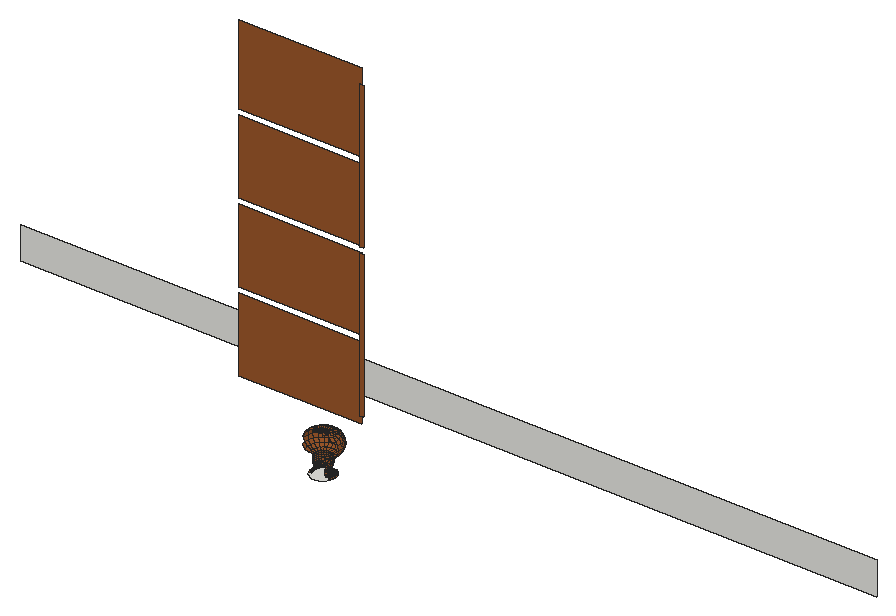
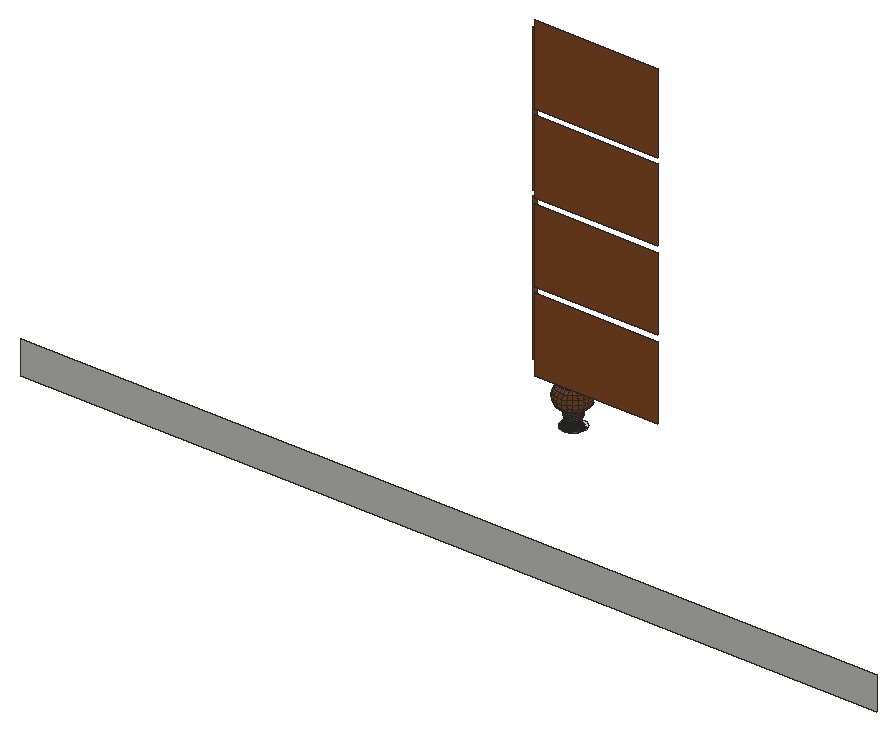
# SketchUp Ruby script. Lengths in inches.
U = 1.inch
M = Sketchup.active_model
def pt(a) = Geom::Point3d.new(a.map { |v| v * U })
def face(e, loops, mat)
  f = e.add_face(loops[0].map { |a| pt(a) })
  loops[1..].each { |l| e.add_face(l.map { |a| pt(a) }).erase! }
  f.material = f.back_material = mat if mat
  f
end
# faces: each face lists its corners as indices into pts; further lists are holes
def faces(e, pts, list, mat = nil) = list.each { |f| face(e, (f[0].is_a?(Array) ? f : [f]).map { |l| l.map { |i| pts[i] } }, mat) }
# xy, xz, yz: faces in a plane at the given z, y or x. An outline is a flat list of corners, or four numbers for a rectangle; further outlines are holes
def ring(l) = l.size == 4 ? [[l[0], l[1]], [l[2], l[1]], [l[2], l[3]], [l[0], l[3]]] : l.each_slice(2).to_a
def flat(e, list, mat, &to3) = list.each { |f| face(e, (f[0].is_a?(Array) ? f : [f]).map { |l| ring(l).map { |u, v| to3.(u, v) } }, mat) }
def xy(e, z, list, mat = nil) = flat(e, list, mat) { |x, y| [x, y, z] }
def xz(e, y, list, mat = nil) = flat(e, list, mat) { |x, z| [x, y, z] }
def yz(e, x, list, mat = nil) = flat(e, list, mat) { |y, z| [x, y, z] }
def lines(e, pts, list) = list.each { |a, b| e.add_line(pt(pts[a]), pt(pts[b])) }
# prism: a flat outline (further loops are holes) pulled along v
def prism(e, loops, v, mat = nil)
  f = face(e, loops, mat); d = Geom::Vector3d.new(v.map { |x| x * U })
  f.pushpull(f.normal.samedirection?(d) ? d.length : -d.length)
end
def box(e, o, s, mat = nil) = prism(e, [[o, [o[0] + s[0], o[1], o[2]], [o[0] + s[0], o[1] + s[1], o[2]], [o[0], o[1] + s[1], o[2]]]], [0, 0, s[2]], mat)
def at(x, y, z, deg = 0) = Geom::Transformation.translation(pt([x, y, z])) * Geom::Transformation.rotation(ORIGIN, Z_AXIS, deg.degrees)
def axes(o, x, y, z) = Geom::Transformation.new([*x, 0, *y, 0, *z, 0, *pt(o).to_a, 1])
def part(name) = M.definitions.add(name)
# library, detail: a bought-in or finely detailed component or shape, given as its bounding box
def library(name, o, s) = part(name).tap { |d| box(d.entities, o, s) }
def detail(e, o, s) = box(e.add_group.entities, o, s)
def put(e, d, t, mat = nil) = e.add_instance(d, t).tap { |i| i.material = mat if mat }
def group(e, t, mat = nil) = e.add_group.tap { |g| g.transformation = t; g.material = mat if mat }.entities
root = M.entities
M.materials.add("[Wood Cherry Original]").color = [152, 86, 42]
xy(root,6,[[197.18,64.59,197.74,64.59,198.28,64.73,198.76,65.01,199.16,65.4,199.4375,65.89,199.59,66.42,199.59,66.98,199.44,67.52,199.17,68.01,198.77,68.4,198.29,68.69,197.75,68.83,197.19,68.83,196.65,68.69,196.17,68.41,195.77,68.02,195.49,67.54,195.35,67,195.34,66.44,195.49,65.9,195.76,65.42,196.16,65.02,196.64,64.74]])
xy(root,6,[[199.4375,65.89,199.59,66.42,199.44,66.45,199.3,65.94],[195.49,65.9,195.625,65.96,195.49,66.46,195.34,66.44],[199.59,66.42,199.59,66.98,199.4375,66.96,199.44,66.45],[195.34,66.44,195.49,66.46,195.5,66.98,195.35,67],[199.4375,66.96,199.59,66.98,199.44,67.52,199.3,67.47],
  [195.5,66.98,195.63,67.48,195.49,67.54,195.35,67],[199.3,67.47,199.44,67.52,199.17,68.01,199.05,67.92],[195.63,67.48,195.89,67.93,195.77,68.02,195.49,67.54],[199.05,67.92,199.17,68.01,198.77,68.4,198.68,68.28],[195.89,67.93,196.26,68.29,196.17,68.41,195.77,68.02],
  [198.68,68.28,198.77,68.4,198.29,68.69,198.23,68.55],[196.26,68.29,196.71,68.55,196.65,68.69,196.17,68.41],[196.71,68.55,197.21,68.68,197.19,68.83,196.65,68.69],[198.23,68.55,198.29,68.69,197.75,68.83,197.73,68.68],[197.21,68.68,197.73,68.68,197.75,68.83,197.19,68.83]],"[Wood Cherry Original]")
xz(root,67.9,[[197.3125,6.79,197.63,6.94]],"[Wood Cherry Original]")
xz(root,68.21,[[197.27,8.1,197.67,8.4]],"[Wood Cherry Original]")
xz(root,69.11,[[202.15,16.08,202.9,42.58],[202.15,43.58,202.9,70.08]],"[Wood Cherry Original]")
xz(root,70.11,[[179.35,14.08,201.81,27.58],[179.35,28.58,201.81,42.08],[179.35,43.08,201.81,56.58],[179.35,57.58,201.81,72.08]],"[Wood Cherry Original]")
xz(root,96.25,[[118.75,0,274.48,6]])
yz(root,195.97,[[66.52,8.1,66.52,8.4,66.92,8.4,66.91,8.1]],"[Wood Cherry Original]")
yz(root,196.27,[[66.56,6.79,66.875,6.94]],"[Wood Cherry Original]")
yz(root,198.66,[[66.55,6.79,66.86,6.94]],"[Wood Cherry Original]")
yz(root,198.96,[[66.51,8.1,66.9,8.4]],"[Wood Cherry Original]")
p = [[199.16,66,6.03],[199.3,65.94,6],[199.44,66.45,6],[199.29,66.47,6.03],[195.64,66.48,6.03],[195.49,66.46,6],
  [195.625,65.96,6],[195.76,66.02,6.03],[195.78,66.5,6.08],[195.9,66.07,6.08],[199.03,66.06,6.08],[199.15,66.48,6.08],
  [199.4375,66.96,6],[199.29,66.95,6.03],[195.64,66.96,6.03],[195.5,66.98,6],[195.78,66.94,6.08],[199.15,66.93,6.08],
  [195.9,67.37,6.08],[195.77,67.42,6.03],[199.17,67.41,6.03],[199.04,67.36,6.08],[199.3,67.47,6],[195.63,67.48,6],
  [196.01,67.84,6.03],[195.89,67.93,6],[196.125,67.75,6.08],[198.93,67.83,6.03],[198.82,67.74,6.08],[199.05,67.92,6],
  [198.59,68.17,6.03],[198.5,68.05,6.08],[196.35,68.18,6.03],[196.26,68.29,6],[196.4375,68.0625,6.08],[198.68,68.28,6],
  [196.82,68.28,6.08],[196.77,68.41,6.03],[198.18,68.41,6.03],[198.12,68.28,6.08],[196.71,68.55,6],[198.23,68.55,6],
  [197.25,68.4,6.08],[197.23,68.54,6.03],[197.71,68.53,6.03],[197.69,68.39,6.08],[197.21,68.68,6],[197.73,68.68,6],
  [195.91,66.51,6.16],[196.02,66.12,6.16],[198.91,66.11,6.16],[199.02,66.5,6.16],[195.91,66.92,6.16],[199.02,66.91,6.16],
  [196.02,67.32,6.16],[198.91,67.31,6.16],[196.23,67.67,6.16],[198.71,67.66,6.16],[196.52,67.96,6.16],[198.42,67.95,6.16],
  [196.87,68.16,6.16],[198.07,68.16,6.16],[197.27,68.27,6.16],[197.68,68.26,6.16],[196.125,66.16,6.25],[196.22,65.76,6.16],
  [196.3125,65.83,6.25],[196.03,66.53,6.25],[198.8,66.15,6.25],[198.9,66.52,6.25],[196.03,66.91,6.25],[198.9,66.9,6.25],
  [196.13,67.27,6.25],[198.81,67.26,6.25],[196.32,67.6,6.25],[198.62,67.59,6.25],[196.59,67.87,6.25],[198.35,67.86,6.25],
  [196.92,68.05,6.25],[198.03,68.05,6.25],[197.28,68.15,6.25],[197.66,68.15,6.25],[196.21,66.2,6.37],[196.39,65.89,6.37],
  [198.54,65.88,6.37],[198.61,65.82,6.25],[198.71,66.1875,6.37],[196.12,66.54,6.37],[198.81,66.53,6.37],[196.125,66.89,6.37],
  [198.81,66.88,6.37],[196.22,67.24,6.37],[198.72,67.23,6.37],[196.39,67.54,6.37],[198.54,67.53,6.37],[196.65,67.79,6.37],
  [198.29,67.78,6.37],[196.95,67.97,6.37],[197.99,67.96,6.37],[197.29,68.06,6.37],[197.65,68.05,6.37],[196.28,66.23,6.5],
  [196.45,65.9375,6.5],[198.48,65.93,6.5],[198.65,66.22,6.5],[196.2,66.55,6.5],[198.73,66.54,6.5],[196.2,66.88,6.5],
  [198.73,66.875,6.5],[196.29,67.21,6.5],[198.65,67.2,6.5],[196.45,67.49,6.5],[198.48,67.49,6.5],[196.69,67.73,6.5],
  [198.25,67.72,6.5],[196.98,67.9,6.5],[197.96,67.89,6.5],[197.3,67.98,6.5],[197.64,67.98,6.5],[196.33,66.25,6.64],
  [196.49,65.97,6.64],[198.4375,65.96,6.64],[198.6,66.24,6.64],[196.25,66.56,6.64],[198.68,66.55,6.64],[198.68,66.87,6.64],
  [196.25,66.88,6.64],[196.33,67.1875,6.64],[198.6,67.18,6.64],[196.49,67.46,6.64],[198.44,67.46,6.64],[196.72,67.6875,6.64],
  [198.22,67.68,6.64],[197,67.85,6.64],[197.94,67.84,6.64],[197.31,67.93,6.64],[197.63,67.93,6.64],[196.35,66.26,6.79],
  [196.51,65.98,6.79],[198.42,65.98,6.79],[198.57,66.25,6.79],[196.27,66.56,6.79],[198.66,66.55,6.79],[198.66,66.86,6.79],
  [196.27,66.875,6.79],[196.36,67.18,6.79],[198.58,67.17,6.79],[196.51,67.45,6.79],[198.42,67.44,6.79],[196.74,67.67,6.79],
  [198.2,67.66,6.79],[197.01,67.82,6.79],[197.93,67.82,6.79],[197.3125,67.9,6.79],[197.63,67.9,6.79],[196.35,66.26,6.94],
  [196.51,65.98,6.94],[198.42,65.98,6.94],[198.57,66.25,6.94],[198.66,66.55,6.94],[196.27,66.56,6.94],[196.36,67.18,6.94],
  [196.27,66.875,6.94],[198.66,66.86,6.94],[198.58,67.17,6.94],[196.51,67.45,6.94],[198.42,67.44,6.94],[196.74,67.67,6.94],
  [198.2,67.66,6.94],[197.01,67.82,6.94],[197.93,67.82,6.94],[197.3125,67.9,6.94],[197.63,67.9,6.94],[196.33,66.25,7.09],
  [196.49,65.97,7.09],[198.4375,65.96,7.09],[198.6,66.24,7.09],[196.25,66.56,7.09],[198.68,66.55,7.09],[198.68,66.87,7.09],
  [196.25,66.88,7.09],[196.33,67.1875,7.09],[198.6,67.18,7.09],[196.49,67.46,7.09],[198.44,67.46,7.09],[196.72,67.69,7.09],
  [198.22,67.68,7.09],[197,67.85,7.09],[197.94,67.85,7.09],[197.31,67.93,7.09],[197.63,67.93,7.09],[196.28,66.23,7.23],
  [196.45,65.9375,7.23],[198.48,65.93,7.23],[198.65,66.22,7.23],[196.2,66.55,7.23],[198.73,66.54,7.23],[196.2,66.88,7.23],
  [198.74,66.875,7.23],[196.28,67.21,7.23],[198.65,67.2,7.23],[196.45,67.5,7.23],[198.48,67.49,7.23],[196.69,67.73,7.23],
  [198.25,67.72,7.23],[196.98,67.9,7.23],[197.96,67.89,7.23],[197.3,67.98,7.23],[197.64,67.98,7.23],[196.18,66.18,7.51],
  [196.36,65.87,7.51],[198.57,65.86,7.51],[198.75,66.17,7.51],[196.09,66.54,7.51],[198.84,66.53,7.51],[196.09,66.9,7.51],
  [198.85,66.89,7.51],[196.18,67.25,7.51],[198.75,67.24,7.51],[196.36,67.5625,7.51],[198.57,67.55,7.51],[196.62,67.82,7.51],
  [198.32,67.8125,7.51],[196.9375,68,7.51],[198,68,7.51],[197.29,68.09,7.51],[197.65,68.09,7.51],[196.11,66.16,7.8],
  [196.3,65.82,7.8],[198.625,65.8125,7.8],[198.82,66.15,7.8],[198.92,66.51,7.8],[196.01,66.53,7.8],[196.01,66.91,7.8],
  [198.92,66.9,7.8],[196.11,67.28,7.8],[198.82,67.27,7.8],[196.3,67.61,7.8],[198.63,67.6,7.8],[196.58,67.88,7.8],
  [198.36,67.87,7.8],[196.91,68.07,7.8],[198.03,68.07,7.8],[197.28,68.17,7.8],[197.66,68.17,7.8],[196.07,66.14,8.1],
  [196.27,65.8,8.1],[198.66,65.79,8.1],[198.86,66.13,8.1],[195.97,66.52,8.1],[198.96,66.51,8.1],[195.97,66.91,8.1],
  [198.96,66.9,8.1],[196.08,67.29,8.1],[198.86,67.28,8.1],[196.27,67.63,8.1],[198.66,67.625,8.1],[196.55,67.91,8.1],
  [198.39,67.9,8.1],[196.89,68.11,8.1],[198.05,68.1,8.1],[197.27,68.21,8.1],[197.67,68.21,8.1],[195.97,66.52,8.4],
  [196.07,66.14,8.4],[198.86,66.13,8.4],[198.96,66.51,8.4],[196.07,67.3,8.4],[195.97,66.92,8.4],[198.96,66.9,8.4],
  [198.86,67.28,8.4],[196.27,67.64,8.4],[198.67,67.625,8.4],[196.55,67.91,8.4],[198.39,67.91,8.4],[196.89,68.11,8.4],
  [198.05,68.11,8.4],[197.27,68.21,8.4],[197.67,68.21,8.4],[196.1,66.15,8.7],[196.26,65.8,8.4],[196.29,65.82,8.7],
  [196,66.53,8.7],[198.83,66.14,8.7],[198.93,66.51,8.7],[196,66.91,8.7],[198.93,66.9,8.7],[196.1,67.28,8.7],
  [198.83,67.27,8.7],[196.3,67.62,8.7],[198.64,67.61,8.7],[196.57,67.89,8.7],[198.37,67.88,8.7],[196.91,68.08,8.7],
  [198.04,68.07,8.7],[197.28,68.18,8.7],[197.66,68.17,8.7],[196.16,66.18,8.99],[196.35,65.86,8.99],[198.58,65.85,8.99],
  [198.63,65.81,8.7],[198.76,66.17,8.99],[198.86,66.52,8.99],[196.07,66.53,8.99],[196.07,66.9,8.99],[198.86,66.89,8.99],
  [196.17,67.26,8.99],[198.77,67.24,8.99],[198.58,67.5625,8.99],[196.35,67.57,8.99],[196.61,67.83,8.99],[198.33,67.82,8.99],
  [196.93,68.01,8.99],[198.01,68.01,8.99],[197.29,68.11,8.99],[197.65,68.1,8.99],[195.375,66.45,9.21],[195.52,65.91,9.21],
  [199.41,65.9,9.21],[199.55,66.43,9.21],[195.375,67,9.21],[199.56,66.98,9.21],[195.52,67.53,9.21],[199.42,67.51,9.21],
  [199.14,67.99,9.21],[195.8,68,9.21],[196.1875,68.39,9.21],[198.76,68.38,9.21],[196.67,68.66,9.21],[198.28,68.66,9.21],
  [197.2,68.8,9.21],[197.75,68.8,9.21],[194.8,66.37,9.66],[194.98,65.69,9.66],[199.94,65.67,9.66],[200.13,66.35,9.66],
  [194.8,67.07,9.66],[200.13,67.05,9.66],[194.99,67.75,9.66],[199.95,67.73,9.66],[195.34,68.36,9.66],[199.6,68.34,9.66],
  [195.84,68.85,9.66],[199.11,68.84,9.66],[196.45,69.2,9.66],[198.5,69.19,9.66],[197.125,69.38,9.66],[197.83,69.375,9.66],
  [194.42,66.32,10.28],[194.63,65.55,10.28],[194.43,67.125,10.28],[200.51,66.3,10.28],[200.51,67.1,10.28],[194.64,67.9,10.28],
  [200.3,67.875,10.28],[195.04,68.59,10.28],[199.91,68.57,10.28],[199.34,69.14,10.28],[195.61,69.15,10.28],[198.65,69.54,10.28],
  [196.3,69.55,10.28],[197.08,69.75,10.28],[197.88,69.75,10.28],[194.29,67.14,11],[194.29,66.31,11],[200.64,66.28,11],
  [200.64,67.12,11],[194.51,67.95,11],[200.43,67.93,11],[194.93,68.67,11],[200.01,68.65,11],[195.53,69.26,11],
  [199.42,69.24,11],[198.7,69.66,11],[196.25,69.67,11],[197.9,69.88,11],[197.06,69.89,11],[194.43,67.125,11.72],
  [194.42,66.32,11.72],[200.51,66.3,11.72],[200.51,67.1,11.72],[194.64,67.9,11.72],[200.3,67.875,11.72],[195.04,68.59,11.72],
  [199.91,68.57,11.72],[195.61,69.15,11.72],[199.34,69.14,11.72],[198.65,69.54,11.72],[196.3,69.55,11.72],[197.88,69.75,11.72],
  [197.08,69.75,11.72],[194.8,66.37,12.34],[194.63,65.55,11.72],[194.98,65.69,12.34],[194.8,67.07,12.34],[200.13,66.35,12.34],
  [200.13,67.05,12.34],[194.99,67.75,12.34],[199.95,67.73,12.34],[195.34,68.36,12.34],[199.6,68.34,12.34],[199.11,68.84,12.34],
  [195.84,68.85,12.34],[198.5,69.19,12.34],[196.45,69.2,12.34],[197.125,69.38,12.34],[197.83,69.375,12.34],[195.375,66.45,12.79],
  [195.52,65.91,12.79],[199.41,65.9,12.79],[199.94,65.67,12.34],[199.55,66.43,12.79],[195.375,67,12.79],[199.56,66.98,12.79],
  [195.52,67.53,12.79],[199.42,67.51,12.79],[195.8,68,12.79],[199.14,67.99,12.79],[196.1875,68.39,12.79],[198.76,68.38,12.79],
  [196.67,68.66,12.79],[198.28,68.66,12.79],[197.2,68.8,12.79],[197.75,68.8,12.79],[197.47,66.71,12.67],[197.21,66.09,12.97],
  [197.375,66.05,12.97],[197.55,66.05,12.97],[197.72,66.09,12.97],[197.05,66.18,12.97],[197.87,66.18,12.97],[196.93,66.31,12.97],
  [198,66.3,12.97],[196.84,66.46,12.97],[198.08,66.45,12.97],[196.8,66.63,12.97],[198.13,66.62,12.97],[196.8,66.8,12.97],
  [198.13,66.8,12.97],[196.85,66.97,12.97],[196.93,67.12,12.97],[197.06,67.25,12.97],[197.21,67.33,12.97],[197.38,67.38,12.97],
  [197.56,67.38,12.97],[198.09,66.97,12.97],[198,67.12,12.97],[197.875,67.24,12.97],[197.72,67.33,12.97],[196.07,66.53,13.01],
  [196.16,66.18,13.01],[198.76,66.17,13.01],[198.86,66.52,13.01],[196.07,66.9,13.01],[198.86,66.89,13.01],[196.17,67.26,13.01],
  [198.77,67.24,13.01],[198.58,67.5625,13.01],[196.35,67.57,13.01],[196.61,67.83,13.01],[198.33,67.82,13.01],[196.93,68.01,13.01],
  [198.01,68.01,13.01],[197.29,68.11,13.01],[197.65,68.1,13.01],[196.35,65.86,13.01],[196.61,65.6,13.01],[198.32,65.59,13.01],
  [198.58,65.85,13.01]]
faces(root,p,[[0,1,2,3],[4,5,6,7],[8,4,7,9],[10,0,3,11],[3,2,12,13],[14,15,5,4],[16,14,4,8],[11,3,13,17],
  [18,19,14,16],[17,13,20,21],[13,12,22,20],[19,23,15,14],[24,25,23,19],[26,24,19,18],[21,20,27,28],[20,22,29,27],
  [28,27,30,31],[32,33,25,24],[34,32,24,26],[27,29,35,30],[36,37,32,34],[31,30,38,39],[37,40,33,32],[30,35,41,38],
  [42,43,37,36],[39,38,44,45],[43,46,40,37],[45,44,43,42],[38,41,47,44],[44,47,46,43],[48,8,9,49],[50,10,11,51],
  [52,16,8,48],[51,11,17,53],[54,18,16,52],[53,17,21,55],[56,26,18,54],[55,21,28,57],[58,34,26,56],[57,28,31,59],
  [60,36,34,58],[59,31,39,61],[62,42,36,60],[61,39,45,63],[63,45,42,62],[64,49,65,66],[67,48,49,64],[68,50,51,69],
  [70,52,48,67],[69,51,53,71],[72,54,52,70],[71,53,55,73],[74,56,54,72],[73,55,57,75],[76,58,56,74],[75,57,59,77],
  [78,60,58,76],[77,59,61,79],[80,62,60,78],[81,63,62,80],[79,61,63,81],[82,64,66,83],[84,85,68,86],[87,67,64,82],
  [86,68,69,88],[89,70,67,87],[88,69,71,90],[91,72,70,89],[90,71,73,92],[93,74,72,91],[92,73,75,94],[95,76,74,93],
  [94,75,77,96],[97,78,76,95],[96,77,79,98],[99,80,78,97],[98,79,81,100],[100,81,80,99],[101,82,83,102],[103,84,86,104],
  [105,87,82,101],[104,86,88,106],[107,89,87,105],[106,88,90,108],[109,91,89,107],[108,90,92,110],[111,93,91,109],[110,92,94,112],
  [113,95,93,111],[112,94,96,114],[115,97,95,113],[114,96,98,116],[117,99,97,115],[116,98,100,118],[118,100,99,117],[119,101,102,120],
  [121,103,104,122],[123,105,101,119],[122,104,106,124],[124,106,108,125],[126,107,105,123],[127,109,107,126],[125,108,110,128],[129,111,109,127],
  [128,110,112,130],[131,113,111,129],[130,112,114,132],[133,115,113,131],[132,114,116,134],[135,117,115,133],[134,116,118,136],[136,118,117,135],
  [137,119,120,138],[139,121,122,140],[141,123,119,137],[140,122,124,142],[142,124,125,143],[144,126,123,141],[145,127,126,144],[143,125,128,146],
  [147,129,127,145],[146,128,130,148],[149,131,129,147],[148,130,132,150],[151,133,131,149],[150,132,134,152],[153,135,133,151],[152,134,136,154],
  [154,136,135,153],[155,137,138,156],[157,139,140,158],[158,140,142,159],[160,141,137,155],[161,145,144,162],[163,143,146,164],[165,147,145,161],
  [164,146,148,166],[167,149,147,165],[166,148,150,168],[169,151,149,167],[168,150,152,170],[171,153,151,169],[170,152,154,172],[173,155,156,174],
  [175,157,158,176],[177,160,155,173],[176,158,159,178],[178,159,163,179],[180,162,160,177],[181,161,162,180],[179,163,164,182],[183,165,161,181],
  [182,164,166,184],[185,167,165,183],[184,166,168,186],[187,169,167,185],[186,168,170,188],[189,171,169,187],[188,170,172,190],[190,172,171,189],
  [191,173,174,192],[193,175,176,194],[195,177,173,191],[194,176,178,196],[197,180,177,195],[196,178,179,198],[199,181,180,197],[198,179,182,200],
  [201,183,181,199],[200,182,184,202],[203,185,183,201],[202,184,186,204],[205,187,185,203],[204,186,188,206],[207,189,187,205],[206,188,190,208],
  [208,190,189,207],[209,191,192,210],[211,193,194,212],[213,195,191,209],[212,194,196,214],[215,197,195,213],[214,196,198,216],[217,199,197,215],
  [216,198,200,218],[219,201,199,217],[218,200,202,220],[221,203,201,219],[220,202,204,222],[223,205,203,221],[222,204,206,224],[225,207,205,223],
  [224,206,208,226],[226,208,207,225],[227,209,210,228],[229,211,212,230],[230,212,214,231],[232,213,209,227],[233,215,213,232],[231,214,216,234],
  [235,217,215,233],[234,216,218,236],[237,219,217,235],[236,218,220,238],[239,221,219,237],[238,220,222,240],[241,223,221,239],[240,222,224,242],
  [243,225,223,241],[242,224,226,244],[244,226,225,243],[245,227,228,246],[247,229,230,248],[249,232,227,245],[248,230,231,250],[251,233,232,249],
  [250,231,234,252],[253,235,233,251],[252,234,236,254],[255,237,235,253],[254,236,238,256],[257,239,237,255],[256,238,240,258],[259,241,239,257],
  [258,240,242,260],[261,243,241,259],[260,242,244,262],[262,244,243,261],[263,249,245,264],[265,248,250,266],[267,253,251,268],[269,252,254,270],
  [271,255,253,267],[270,254,256,272],[273,257,255,271],[272,256,258,274],[275,259,257,273],[274,258,260,276],[277,261,259,275],[276,260,262,278],
  [279,264,280,281],[282,263,264,279],[283,265,266,284],[285,268,263,282],[284,266,269,286],[287,267,268,285],[286,269,270,288],[289,271,267,287],
  [288,270,272,290],[291,273,271,289],[290,272,274,292],[293,275,273,291],[292,274,276,294],[295,277,275,293],[294,276,278,296],[296,278,277,295],
  [297,279,281,298],[299,300,283,301],[301,283,284,302],[303,282,279,297],[304,285,282,303],[302,284,286,305],[306,287,285,304],[305,286,288,307],
  [307,288,290,308],[309,289,287,306],[310,291,289,309],[308,290,292,311],[312,293,291,310],[311,292,294,313],[314,295,293,312],[313,294,296,315],
  [315,296,295,314],[316,303,297,317],[318,301,302,319],[320,304,303,316],[319,302,305,321],[322,306,304,320],[321,305,307,323],[323,307,308,324],
  [325,309,306,322],[326,310,309,325],[324,308,311,327],[328,312,310,326],[327,311,313,329],[330,314,312,328],[329,313,315,331],[331,315,314,330],
  [332,316,317,333],[334,318,319,335],[336,320,316,332],[335,319,321,337],[338,322,320,336],[337,321,323,339],[340,325,322,338],[339,323,324,341],
  [342,326,325,340],[341,324,327,343],[344,328,326,342],[343,327,329,345],[346,330,328,344],[345,329,331,347],[347,331,330,346],[348,332,333,349],
  [350,336,332,348],[351,335,337,352],[353,338,336,350],[352,337,339,354],[355,340,338,353],[354,339,341,356],[356,341,343,357],[358,342,340,355],
  [357,343,345,359],[360,344,342,358],[361,346,344,360],[359,345,347,362],[362,347,346,361],[363,350,348,364],[365,351,352,366],[367,353,350,363],
  [366,352,354,368],[369,355,353,367],[368,354,356,370],[371,358,355,369],[370,356,357,372],[372,357,359,373],[374,360,358,371],[373,359,362,375],
  [376,361,360,374],[375,362,361,376],[377,363,364,378],[379,365,366,380],[381,367,363,377],[380,366,368,382],[383,369,367,381],[382,368,370,384],
  [385,371,369,383],[384,370,372,386],[386,372,373,387],[388,374,371,385],[387,373,375,389],[390,376,374,388],[389,375,376,390],[391,378,392,393],
  [394,377,378,391],[395,379,380,396],[397,381,377,394],[396,380,382,398],[399,383,381,397],[398,382,384,400],[400,384,386,401],[402,385,383,399],
  [401,386,387,403],[404,388,385,402],[405,390,388,404],[403,387,389,406],[406,389,390,405],[407,391,393,408],[409,410,395,411],[412,394,391,407],
  [411,395,396,413],[414,397,394,412],[413,396,398,415],[416,399,397,414],[415,398,400,417],[418,402,399,416],[417,400,401,419],[420,404,402,418],
  [419,401,403,421],[422,405,404,420],[421,403,406,423],[423,406,405,422],[424,425,426],[424,426,427],[424,427,428],[424,429,425],
  [424,428,430],[424,431,429],[424,430,432],[424,433,431],[424,432,434],[424,435,433],[424,434,436],[424,437,435],
  [424,436,438],[424,439,437],[424,440,439],[424,441,440],[424,442,441],[424,443,442],[424,444,443],[424,438,445],
  [424,445,446],[424,446,447],[424,447,448],[424,448,444],[449,407,408,450],[451,409,411,452],[453,412,407,449],[452,411,413,454],
  [455,414,412,453],[454,413,415,456],[456,415,417,457],[458,416,414,455],[459,418,416,458],[457,417,419,460],[461,420,418,459],[460,419,421,462],
  [463,422,420,461],[462,421,423,464],[464,423,422,463],[431,465,466,429],[430,467,468,432],[433,450,465,431],[432,468,451,434],[435,449,450,433],
  [434,451,452,436],[437,453,449,435],[436,452,454,438],[439,455,453,437],[438,454,456,445],[440,458,455,439],[445,456,457,446],[441,459,458,440],
  [446,457,460,447],[442,461,459,441],[447,460,462,448],[443,463,461,442],[448,462,464,444],[444,464,463,443]],"[Wood Cherry Original]")
